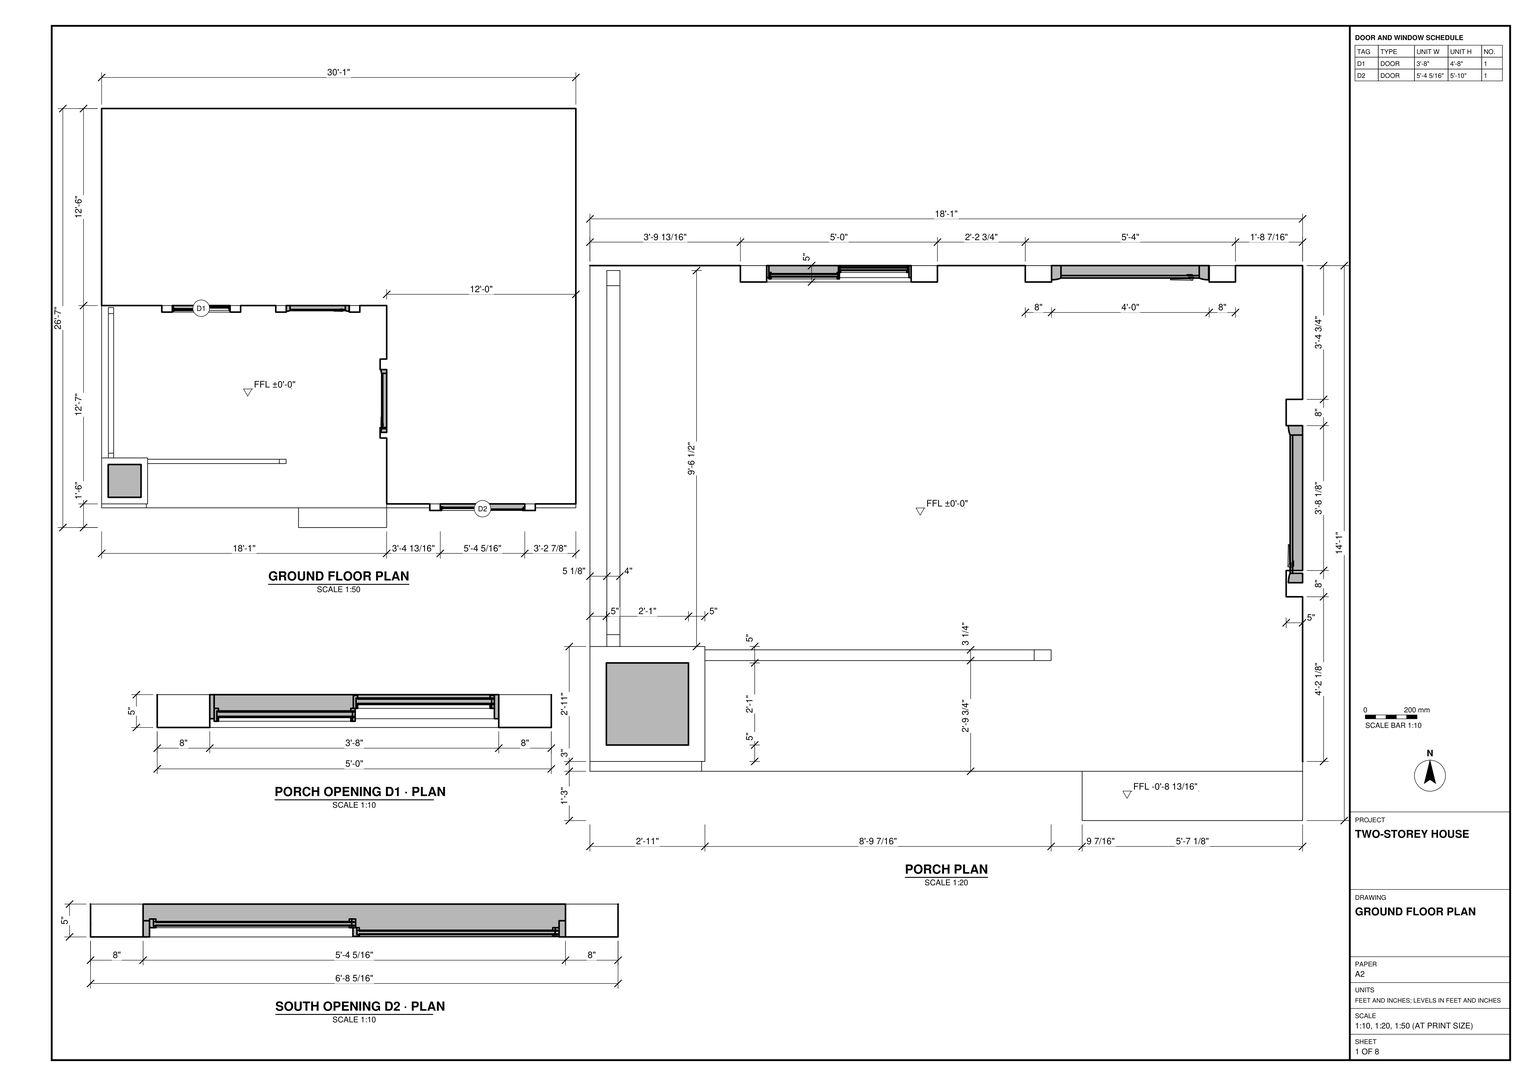
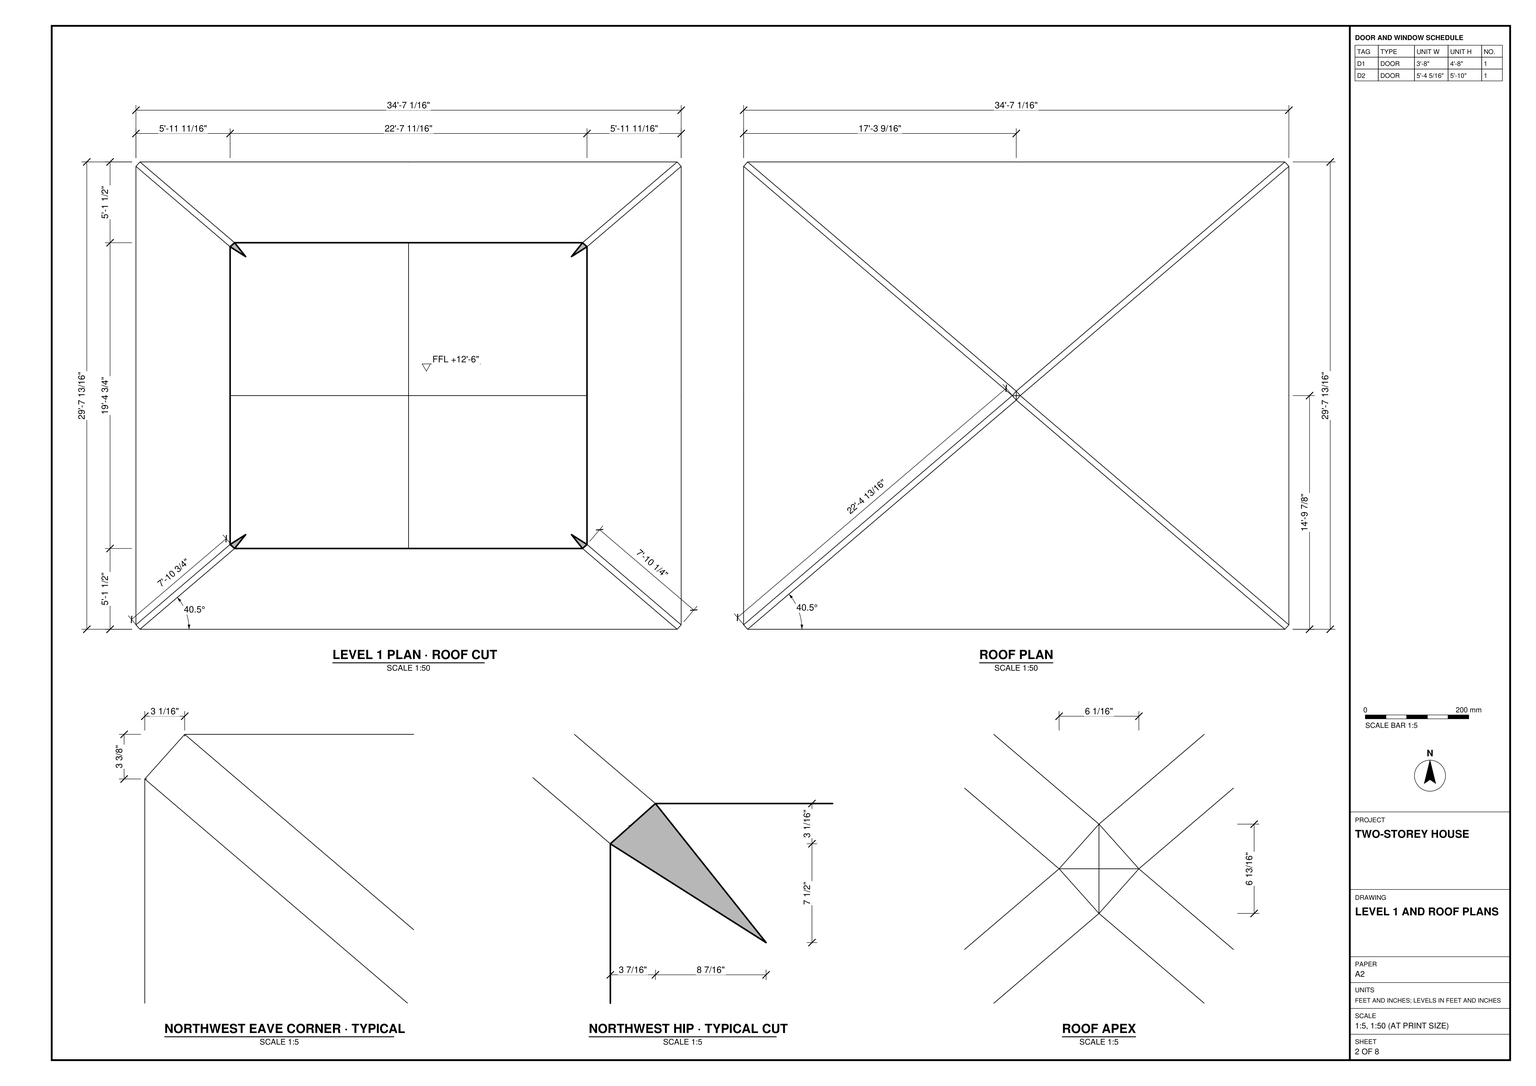
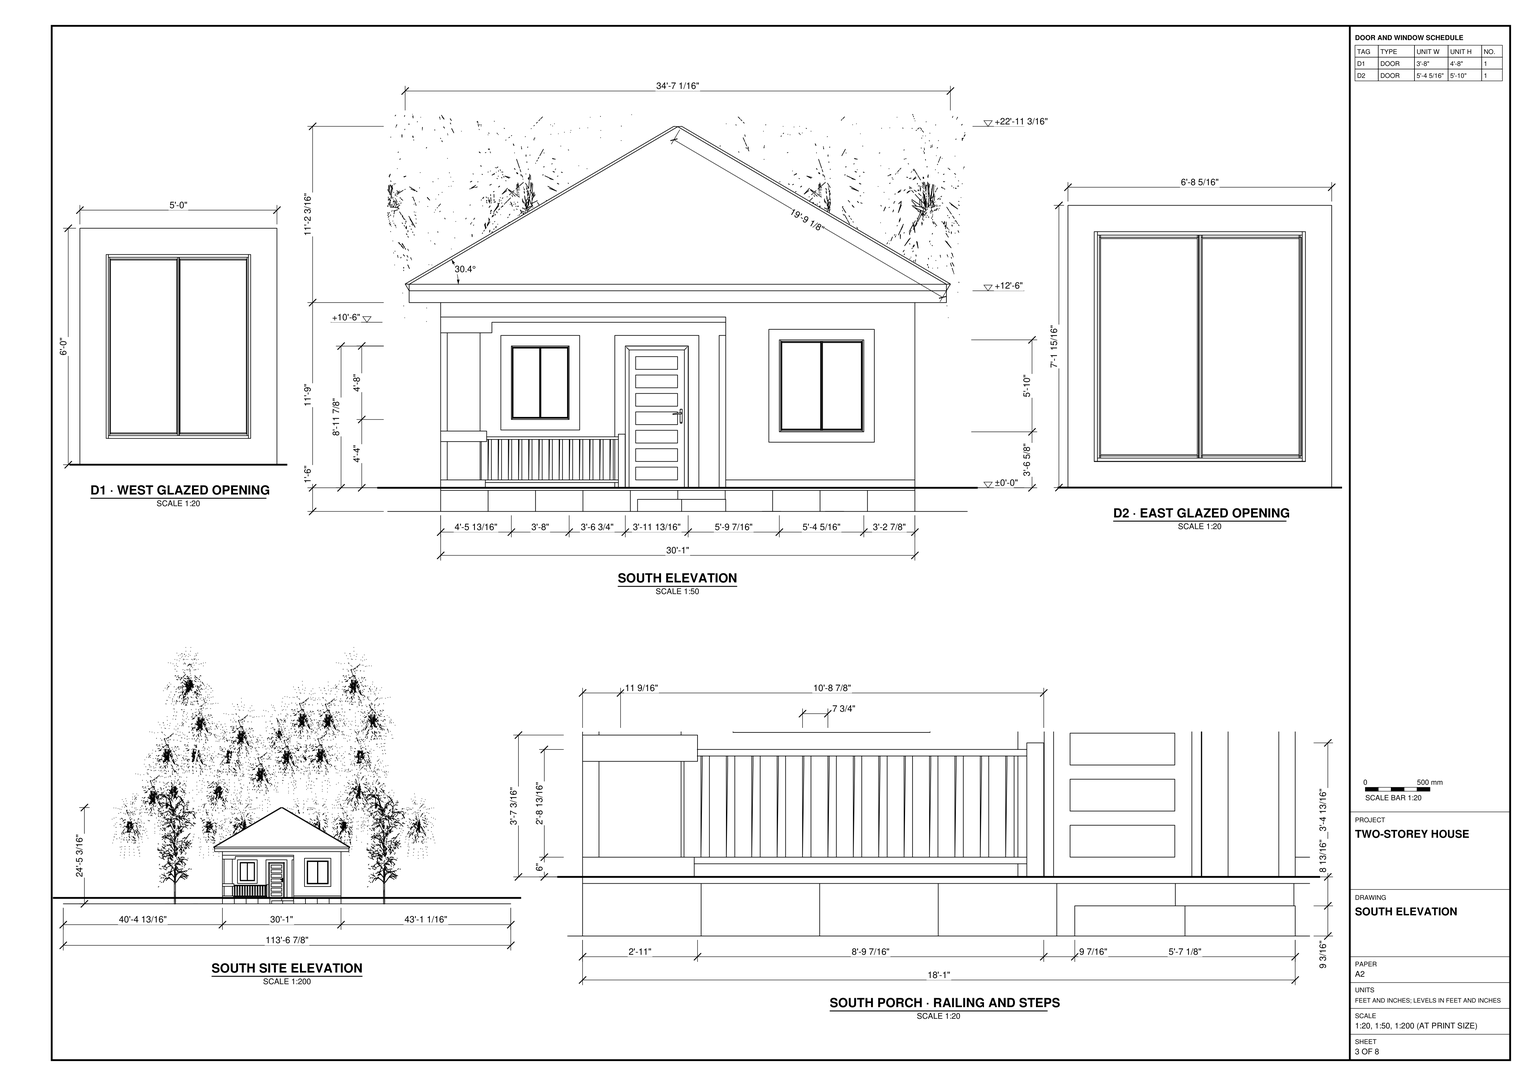
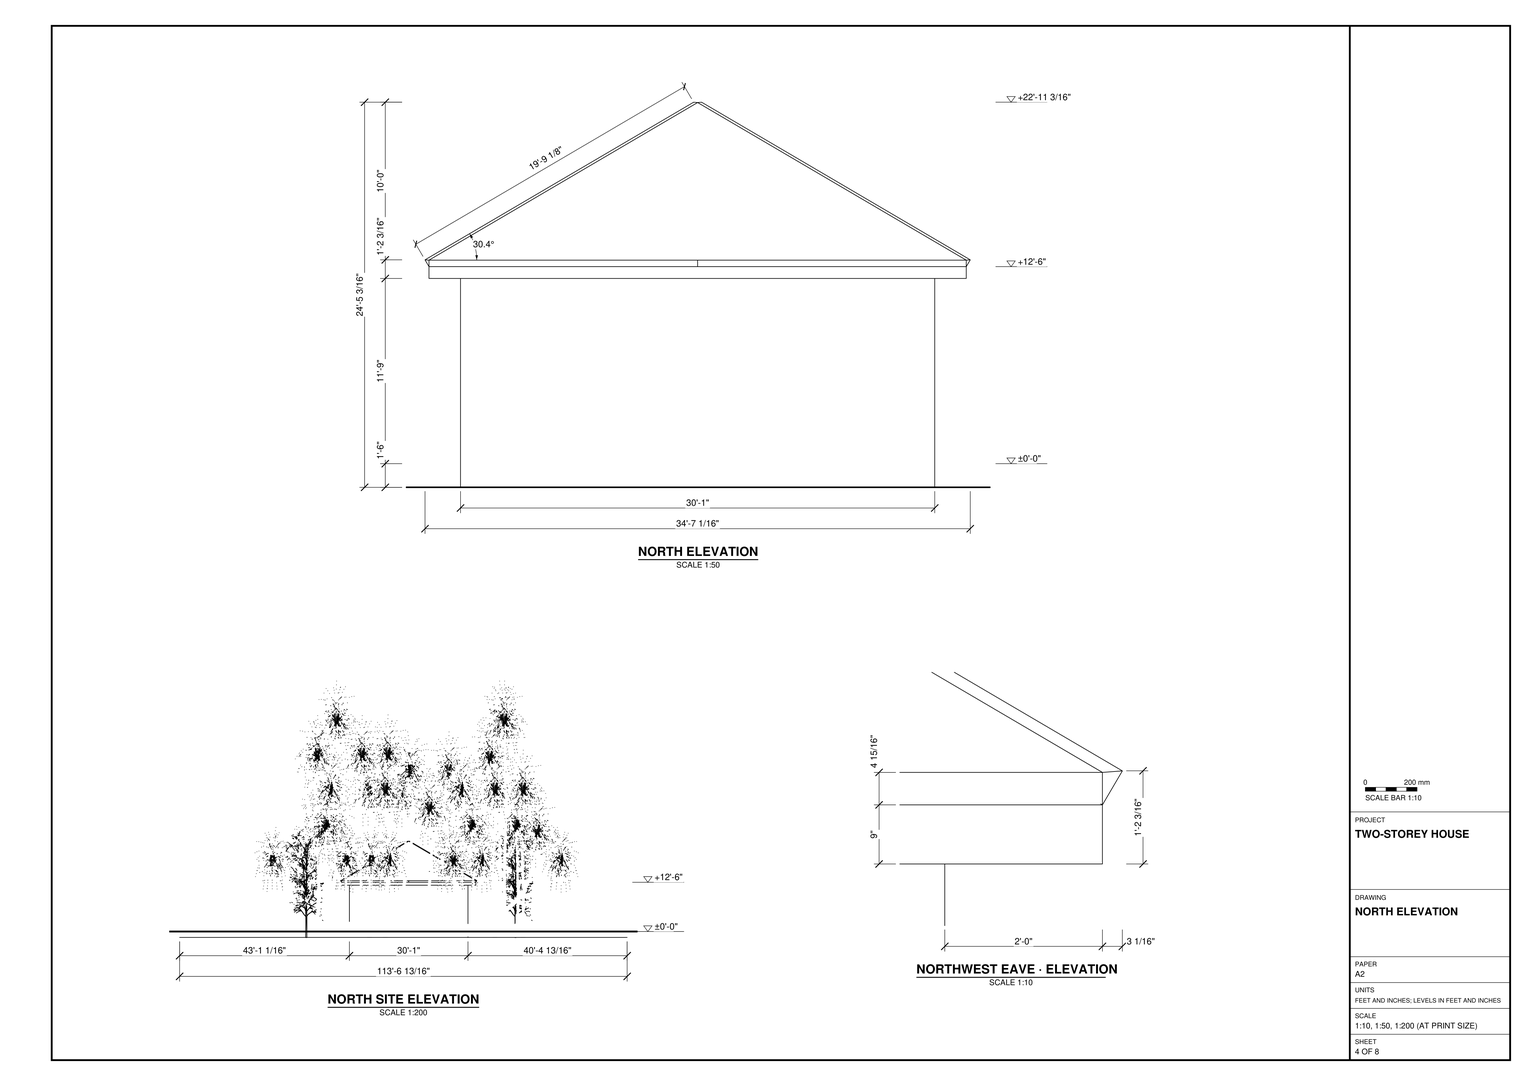
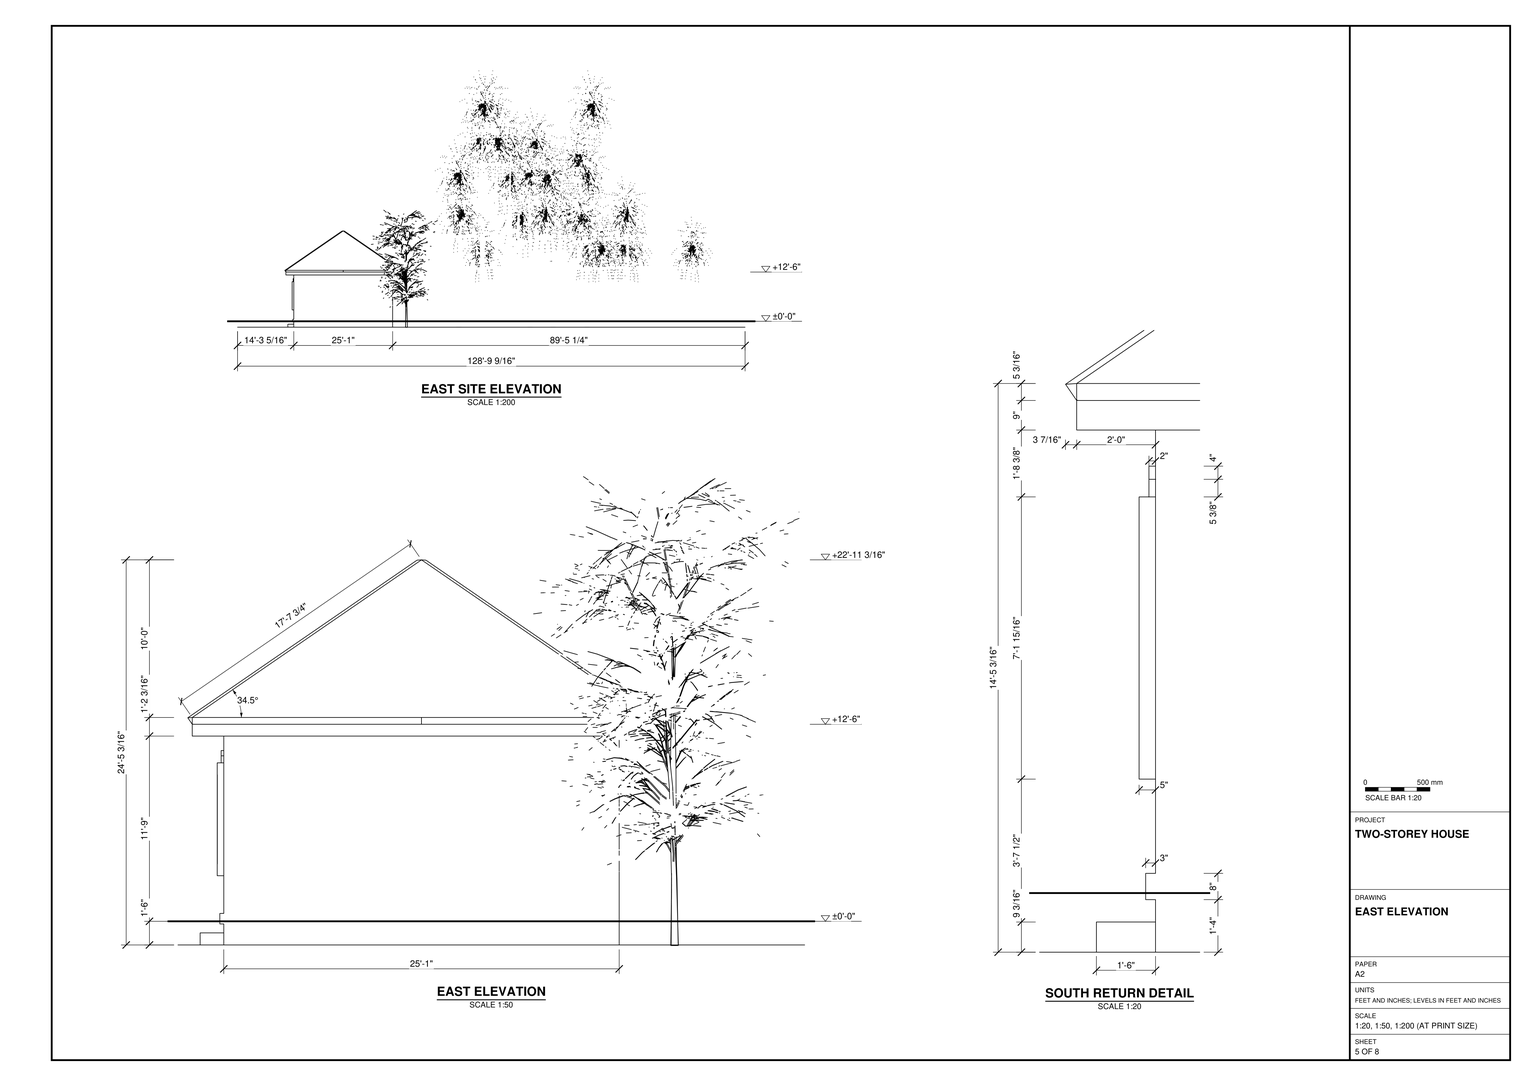
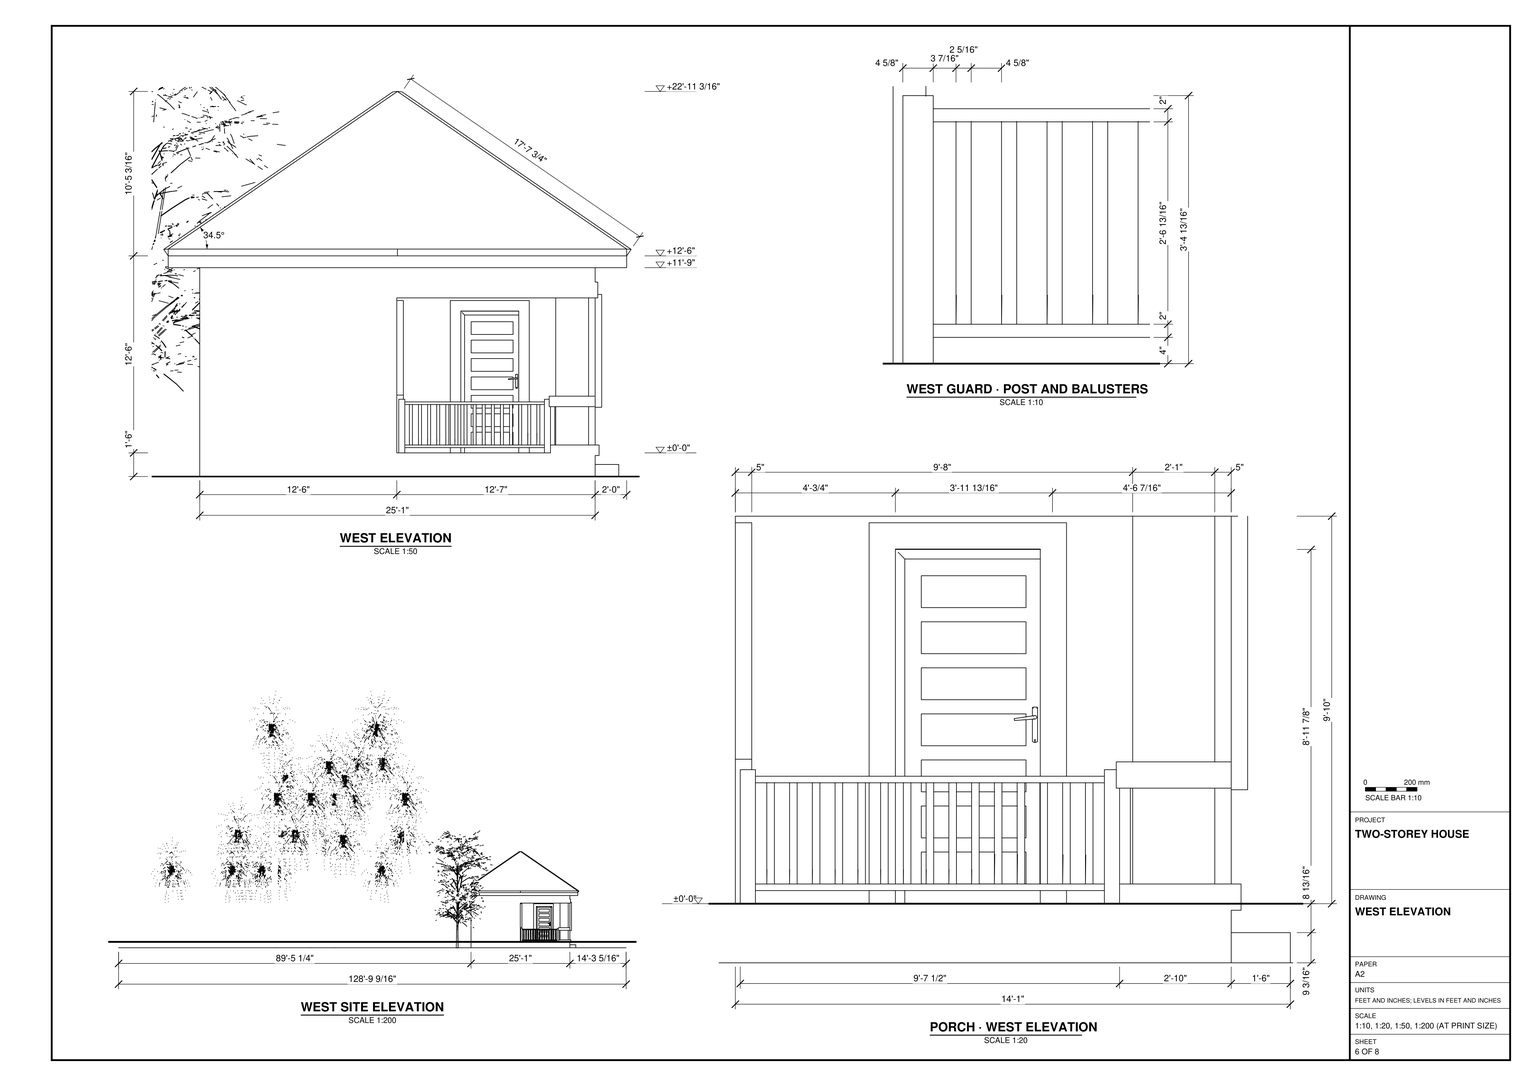
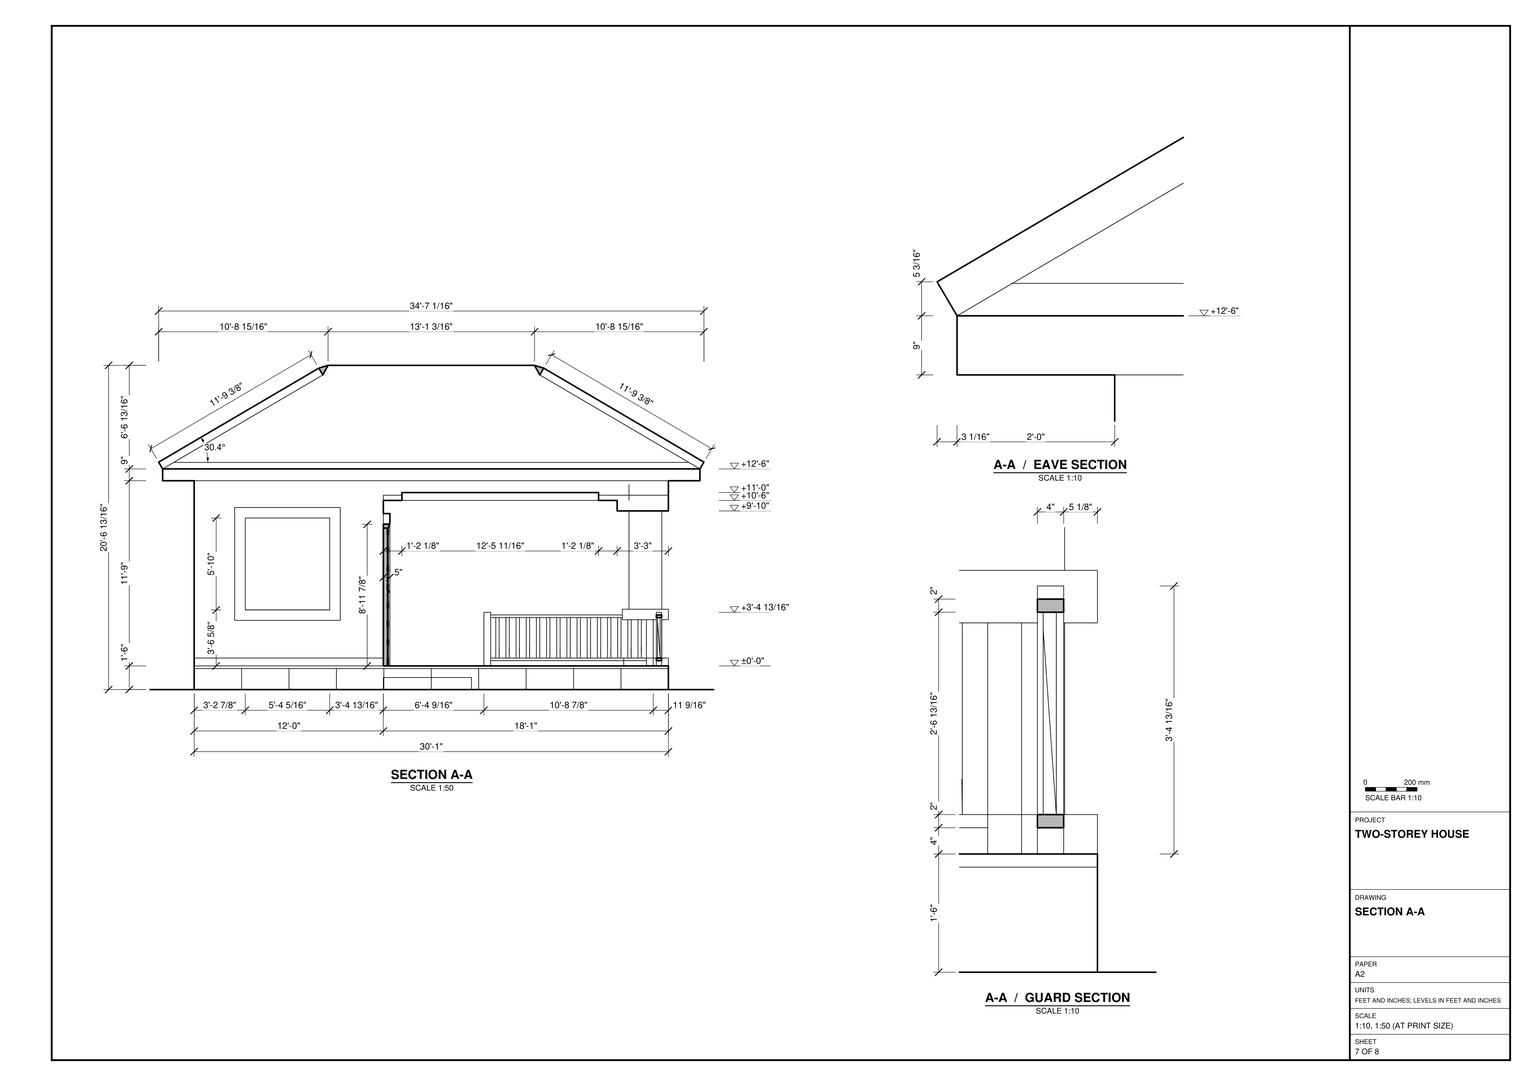
Build the house and its setting in SketchUp from task_files/diagram_01.pdf. Work in feet and inches. The complete model, including the site and planting, measures 113'-6 7/8" along X, 128'-9 9/16" along Y and 65'-6 1/2" along Z. Set the ground floor at ±0'-0" and the upper level at +12'-6".

Use the 30'-1" south frontage to lay out the house on its raised base. Follow the wall thicknesses and opening positions in plan. Recess the porch on the west part of the frontage, leaving the east part enclosed. Model the porch slab, entry steps, square corner support and railing, leaving a clear approach from the steps to the panelled entrance door. Fit the framed, two-panel glazed units into the walls, with the smaller unit at the back of the porch and the larger unit in the projecting south wall.

Use the upper-level roof cut and the roof plan to form four sloping faces that meet at a central apex. Carry the eaves beyond the walls and model the fascia shown in elevation. Include the trees around the house as shown in the site view. Planting, decor and loose items may be represented by any suitable library components.

Keep shell elements such as walls, slabs and roof, and each furniture or joinery piece shown, in separate groups or components. Use components for repeated parts. Save one SketchUp model as output_files/two_storey_house_with_a_recessed_porch_and_hipped_roof.skp.

# SketchUp Ruby script. Lengths in inches.
U = 1.inch
M = Sketchup.active_model
def pt(a) = Geom::Point3d.new(a.map { |v| v * U })
def face(e, loops, mat)
  f = e.add_face(loops[0].map { |a| pt(a) })
  loops[1..].each { |l| e.add_face(l.map { |a| pt(a) }).erase! }
  f.material = f.back_material = mat if mat
  f
end
# faces: each face lists its corners as indices into pts; further lists are holes
def faces(e, pts, list, mat = nil) = list.each { |f| face(e, (f[0].is_a?(Array) ? f : [f]).map { |l| l.map { |i| pts[i] } }, mat) }
# xy, xz, yz: faces in a plane at the given z, y or x. An outline is a flat list of corners, or four numbers for a rectangle; further outlines are holes
def ring(l) = l.size == 4 ? [[l[0], l[1]], [l[2], l[1]], [l[2], l[3]], [l[0], l[3]]] : l.each_slice(2).to_a
def flat(e, list, mat, &to3) = list.each { |f| face(e, (f[0].is_a?(Array) ? f : [f]).map { |l| ring(l).map { |u, v| to3.(u, v) } }, mat) }
def xy(e, z, list, mat = nil) = flat(e, list, mat) { |x, y| [x, y, z] }
def xz(e, y, list, mat = nil) = flat(e, list, mat) { |x, z| [x, y, z] }
def yz(e, x, list, mat = nil) = flat(e, list, mat) { |y, z| [x, y, z] }
def lines(e, pts, list) = list.each { |a, b| e.add_line(pt(pts[a]), pt(pts[b])) }
# prism: a flat outline (further loops are holes) pulled along v
def prism(e, loops, v, mat = nil)
  f = face(e, loops, mat); d = Geom::Vector3d.new(v.map { |x| x * U })
  f.pushpull(f.normal.samedirection?(d) ? d.length : -d.length)
end
def box(e, o, s, mat = nil) = prism(e, [[o, [o[0] + s[0], o[1], o[2]], [o[0] + s[0], o[1] + s[1], o[2]], [o[0], o[1] + s[1], o[2]]]], [0, 0, s[2]], mat)
def at(x, y, z, deg = 0) = Geom::Transformation.translation(pt([x, y, z])) * Geom::Transformation.rotation(ORIGIN, Z_AXIS, deg.degrees)
def axes(o, x, y, z) = Geom::Transformation.new([*x, 0, *y, 0, *z, 0, *pt(o).to_a, 1])
def part(name) = M.definitions.add(name)
# library, detail: a bought-in or finely detailed component or shape, given as its bounding box
def library(name, o, s) = part(name).tap { |d| box(d.entities, o, s) }
def detail(e, o, s) = box(e.add_group.entities, o, s)
def put(e, d, t, mat = nil) = e.add_instance(d, t).tap { |i| i.material = mat if mat }
def group(e, t, mat = nil) = e.add_group.tap { |g| g.transformation = t; g.material = mat if mat }.entities
root = M.entities
M.materials.add("COCOLUMBER1").color = [119, 109, 95]
M.materials.add("Glass_Tinted_Gray").color = [0, 0, 0]
M.materials["Glass_Tinted_Gray"].alpha = 0.125
M.materials.add("Wood_Grain_Dark").color = [94, 66, 25]
M.materials.add("[0049_Beige]").color = [245, 245, 220]
M.materials.add("[0135_DarkGray]").color = [81, 81, 81]
M.materials.add("[Granite Dark Gray]").color = [69, 68, 68]
M.materials.add("[Granite Tile]").color = [155, 148, 143]
M.materials.add("[Grass Dark Green]").color = [106, 157, 55]
M.materials.add("[Grass Light Green]").color = [138, 158, 69]
M.materials.add("[Mirror 02]").color = [229, 229, 229]
M.materials.add("[Roofing Tile Spanish]").color = [138, 64, 36]
M.materials.add("[Stone_Flagstone_Ashlar]").color = [175, 116, 102]
M.materials.add("[Terrazzo Light Blue]").color = [196, 214, 227]
c1 = part("PENTEK_RP Fineline 50S_Sliding_DoorCase_E1")
box(c1.entities,[0,0,0],[1.51,3.66,99.27],"[0135_DarkGray]")
c2 = part("PENTEK_RP Fineline 50S_SlidingDooe_Case_E2")
box(c2.entities,[0,0,0],[96.25,3.66,1.51],"[0135_DarkGray]")
c3 = part("pentek_RP Fineline 50S_SlidingDoor_Case")
put(c3.entities,c1,at(97.76,0,0))
put(c3.entities,c2,at(1.51,0,0))
put(c3.entities,c1,at(0,0,0))
put(c3.entities,c2,at(1.51,0,97.76))
c4 = part("PENTEK_RP Fineline 50S_SlidingDoor_GlazingBead_2")
box(c4.entities,[0,0,0],[0.56,0.59,94.39],"[0135_DarkGray]")
c5 = part("PENTEK_RP Fineline 50S_SlidingDoor_Glass")
box(c5.entities,[0,0,0],[46.58,0.16,94.39],"Glass_Tinted_Gray")
c6 = part("PENTEK_RP Fineline 50S_SlidingDoor_GlazingBead")
box(c6.entities,[0,0,0],[45.47,0.59,0.56],"[0135_DarkGray]")
c7 = part("PENTEK_RP Fineline 50S_SlidingDoor_Leaf_E1")
xy(c7.entities,0,[[0,0,0.93,1.97],[0.93,1.57,1.49,1.97]],"[0135_DarkGray]")
xy(c7.entities,96.25,[[0,0,0.93,0,0.93,1.57,1.49,1.57,1.49,1.97,0,1.97]],"[0135_DarkGray]")
xz(c7.entities,0,[[0,0,0.93,96.25]],"[0135_DarkGray]")
xz(c7.entities,1.57,[[0.93,0,1.49,95.32],[0.93,95.32,1.49,96.25]],"[0135_DarkGray]")
xz(c7.entities,1.97,[[0,0,1.49,96.25]],"[0135_DarkGray]")
yz(c7.entities,0,[[0,0,1.97,96.25]],"[0135_DarkGray]")
yz(c7.entities,0.93,[[0,0,1.57,0.93],[0,0.93,1.57,95.32],[0,95.32,1.57,96.25]],"[0135_DarkGray]")
yz(c7.entities,1.49,[[1.57,0,1.97,95.32],[1.57,95.32,1.97,96.25]],"[0135_DarkGray]")
c8 = part("PENTEK_RP Fineline 50S_SlidingDoor_Leaf_E2")
xy(c8.entities,0,[[0,0,0,1.57,0.56,1.57,0.56,1.97,46.02,1.97,46.02,1.57,46.58,1.57,46.58,0]],"[0135_DarkGray]")
xy(c8.entities,0.93,[[0,0,46.58,1.57]],"[0135_DarkGray]")
xy(c8.entities,1.49,[[0.56,1.57,46.02,1.97]],"[0135_DarkGray]")
xz(c8.entities,0,[[0,0,46.58,0.93]],"[0135_DarkGray]")
xz(c8.entities,1.57,[[0,0,0.56,0.93],[46.02,0,46.58,0.93],[0.56,0.93,46.02,1.49]],"[0135_DarkGray]")
xz(c8.entities,1.97,[[0.56,0,46.02,1.49]],"[0135_DarkGray]")
yz(c8.entities,0,[[0,0,1.57,0.93]],"[0135_DarkGray]")
yz(c8.entities,0.56,[[1.57,0,1.97,0.93],[1.57,0.93,1.97,1.49]],"[0135_DarkGray]")
yz(c8.entities,46.02,[[1.57,0,1.97,0.93],[1.57,0.93,1.97,1.49]],"[0135_DarkGray]")
yz(c8.entities,46.58,[[0,0,1.57,0.93]],"[0135_DarkGray]")
c9 = part("PENTEK_RP Fineline S_SlidingDoor_Leaf1")
put(c9.entities,c4,at(0.93,0,0.93))
put(c9.entities,c4,at(46.96,0,0.93))
put(c9.entities,c5,at(1.49,1.42,0.93))
put(c9.entities,c6,at(1.49,0,0.93))
put(c9.entities,c5,at(1.49,0.59,0.93),"[Terrazzo Light Blue]")
put(c9.entities,c7,at(0,0,0))
put(c9.entities,c7,axes([48.44,0,0],[-1,0,0],[0,1,0],[0,0,1]))
put(c9.entities,c8,axes([0.93,0,96.25],[1,0,0],[0,1,0],[0,0,-1]))
put(c9.entities,c8,at(0.93,0,0))
put(c9.entities,c6,at(1.49,0,94.77))
c10 = part("PENTEK_RP Fineline 50S_SlidingDoor_Leaf2")
put(c10.entities,c5,at(1.49,1.42,0.93))
put(c10.entities,c6,at(1.49,0,94.77))
put(c10.entities,c4,at(46.96,0,0.93))
put(c10.entities,c5,at(1.49,0.59,0.93),"[Mirror 02]")
put(c10.entities,c4,at(0.93,0,0.93))
put(c10.entities,c7,at(0,0,0))
put(c10.entities,c7,axes([48.44,0,0],[-1,0,0],[0,1,0],[0,0,1]))
put(c10.entities,c6,at(1.49,0,0.93))
put(c10.entities,c8,axes([0.93,0,96.25],[1,0,0],[0,1,0],[0,0,-1]))
put(c10.entities,c8,at(0.93,0,0))
c11 = part("PENTEK - Slimmest Steel Sliding Door / Window\#1")
put(c11.entities,c3,at(0,-1.88,-0.09))
put(c11.entities,c9,at(1.51,-2.27,1.42))
put(c11.entities,c10,at(49.32,-0.3,1.42))
c12 = library("Untitled (4)",[17.32,30.71,0],[35.44,8.12,78.74])
c13 = part("railing post")
xy(c13.entities,0,[[0,0,2,2]],"Wood_Grain_Dark")
xy(c13.entities,31,[[0,0,2,0,2,2,0.3125,2]],"Wood_Grain_Dark")
xz(c13.entities,0,[[0,0,2,31]],"Wood_Grain_Dark")
xz(c13.entities,2,[[0,0,0.3125,28.1875,0.3125,31,2,31,2,0]],"Wood_Grain_Dark")
yz(c13.entities,2,[[0,0,2,31]],"Wood_Grain_Dark")
p = [[0.3125,2,28.1875],[0,2,0],[0,0,0],[0,0,31],[0.3125,2,31]]
faces(c13.entities,p,[[0,1,2],[0,2,3,4]],"Wood_Grain_Dark")
c14 = part("cgb5189+Railing+sketch+up")
put(c14.entities,c13,at(60.61,35.39,6))
put(c14.entities,c13,at(66.61,35.39,6))
put(c14.entities,c13,at(72.61,35.39,6))
put(c14.entities,c13,at(78.61,35.39,6))
put(c14.entities,c13,at(84.61,35.39,6))
put(c14.entities,c13,at(90.61,35.39,6))
put(c14.entities,c13,at(96.61,35.39,6))
put(c14.entities,c13,at(102.61,35.39,6))
put(c14.entities,c13,at(54.61,35.39,6))
put(c14.entities,c13,at(48.61,35.39,6))
put(c14.entities,c13,at(42.61,35.39,6))
put(c14.entities,c13,at(36.61,35.39,6))
put(c14.entities,c13,at(30.61,35.39,6))
put(c14.entities,c13,at(24.61,35.39,6))
put(c14.entities,c13,at(18.61,35.39,6))
g1 = group(c14.entities,at(11.61,34.27,0))
box(g1,[0,0,0],[4,4,40.8125],"Wood_Grain_Dark")
g2 = group(c14.entities,at(15.61,34.27,4))
box(g2,[0,0,0],[92,4,2],"Wood_Grain_Dark")
g3 = group(c14.entities,at(15.61,34.27,36.8125))
xy(g3,0,[[0,0,92,4]],"Wood_Grain_Dark")
xy(g3,2,[[0,0,92,4]],"Wood_Grain_Dark")
xz(g3,0,[[0,0,92,2]],"Wood_Grain_Dark")
xz(g3,4,[[0,0,92,2]],"Wood_Grain_Dark")
yz(g3,0,[[0,0,4,2]])
yz(g3,92,[[0,0,4,2]])
g4 = group(c14.entities,at(107.61,34.27,0))
box(g4,[0,0,0],[4,4,40.8125],"Wood_Grain_Dark")
c15 = library("Palm frond",[-21.27,-0.38,-4.44],[74.64,151.68,26.05])
c16 = part("Palm frond cluster")
put(c16.entities,c15,axes([98.98,59.12,-6.6],[-0.57786,0.81614,0],[-0.81614,-0.57786,0],[0,0,1.8876]))
put(c16.entities,c15,axes([105.83,88.13,9.87],[-0.67944,-0.73373,0],[0.7249,-0.67126,-0.15471],[0.21427,-0.19842,1.86487]))
put(c16.entities,c15,axes([73.46,76.73,-6.83],[1,0,0],[0,0.99443,-0.10543],[0,0.19901,1.87708]))
c17 = part("Palm tree")
put(c17.entities,c15,axes([108.09,116.23,112.23],[0.60444,0.79634,0.02211],[-0.38669,0.31755,-0.86581],[-0.57427,0.42444,0.41215]))
put(c17.entities,c15,axes([136.99,132.05,110.62],[-0.9152,-0.38852,0.10706],[0.08408,-0.44389,-0.89213],[0.32496,-0.66577,0.36188]))
put(c17.entities,c15,axes([122.18,113.8,111.54],[0.08804,0.99481,0.05098],[-0.50379,0.08862,-0.85927],[-0.70852,0.0412,0.41966]))
put(c17.entities,c15,axes([127.99,125.91,114.12],[-0.30715,0.21543,0.04369],[-0.00716,-0.23041,1.0858],[0.26841,0.36655,0.07955]))
put(c17.entities,c15,axes([103.59,126.54,118.32],[0.96893,0.24682,0.01605],[-0.22321,0.84461,0.48663],[0.20112,-0.89679,1.64874]))
put(c17.entities,c15,axes([132.625,118.58,110.86],[-0.79198,0.60227,0.10017],[-0.36651,-0.33776,-0.86694],[-0.4026,-0.59638,0.40255]))
put(c17.entities,c15,axes([132.69,143.375,115.86],[-0.48474,-0.87071,0.083],[0.68927,-0.43869,-0.5766],[1.01639,-0.4196,1.53425]))
put(c17.entities,c16,axes([128.89,9.89,132.21],[0.59014,0.791,-0.16144],[-0.79634,0.60321,0.04452],[0.1326,0.10229,0.98588]))
put(c17.entities,c15,axes([110.58,141.22,117.1],[0.63855,-0.76931,0.0202],[0.63758,0.51415,-0.57371],[0.8135,0.71582,1.54559]))
put(c17.entities,c15,axes([124.78,146.64,115.88],[-0.11221,-0.99112,0.07129],[0.92652,-0.13028,-0.35296],[0.67787,0.04993,1.76097]))
put(c17.entities,c15,axes([122.51,149.42,117.04],[0.39103,-0.91975,0.03404],[0.19966,0.04866,-0.97866],[0.74078,0.32113,0.1671]))
put(c17.entities,c15,axes([109.625,140.35,117.99],[0.86054,-0.50891,0.02211],[0.4462,0.77402,0.44921],[-0.46382,-0.71105,1.68592]))
put(c17.entities,c15,axes([116.71,128.1875,118.1],[0.61604,-0.07661,0.00027],[0.03235,0.25679,-0.96593],[0.09819,0.79033,0.2134]),"COCOLUMBER1")
put(c17.entities,c15,axes([106.79,121.78,118.63],[0.90526,0.41496,-0.09122],[-0.38356,0.70587,-0.59551],[-0.34491,1.08363,1.50659]))
put(c17.entities,c15,axes([127.38,115.49,111.15],[-0.41996,0.90406,0.07938],[-0.48716,-0.15078,-0.8602],[-0.63133,-0.32974,0.41534]))
put(c17.entities,c15,axes([126.87,112.82,117.51],[-0.39428,0.9188,-0.01857],[-0.74747,-0.33238,-0.57517],[-1.00919,-0.40185,1.54373]))
put(c17.entities,c15,axes([136.51,114.68,116.54],[-0.8132,0.57038,0.11567],[-0.44883,-0.74115,0.49924],[0.69933,0.66833,1.62089]))
put(c17.entities,c15,axes([139.34,132.85,114.96],[-0.95658,-0.27018,0.10937],[0.1925,-0.86734,-0.45898],[0.41314,-0.78901,1.66428]))
put(c17.entities,c15,axes([114.58,111.42,117.76],[0.273,0.96044,0.05495],[-0.82871,0.20578,0.52048],[0.92224,-0.35418,1.60843]))
put(c17.entities,c16,axes([34.06,50.17,99.19],[1,0,0],[0,0.96593,0.25882],[0,-0.25882,0.96593]))
put(c17.entities,c15,axes([129.57,143.93,113.7],[-0.59821,-0.79634,0.08934],[0.41703,-0.40458,-0.81388],[0.56418,-0.37071,0.47337]))
put(c17.entities,c15,axes([130.72,144.4375,116.95],[-0.38164,-0.91976,0.09155],[0.8496,-0.31006,0.42666],[-0.68716,0.45418,1.6984]))
put(c17.entities,c15,axes([131.04,111.78,119.35],[-0.80044,0.5994,0.00413],[-0.42618,-0.56425,-0.7071],[-0.79563,-1.07169,1.33472]))
put(c17.entities,c15,axes([110.2,144.05,126.35],[0.60643,-0.7943,0.03632],[0.64903,0.52087,0.55448],[-0.86705,-0.59022,1.56936]))
put(c17.entities,c15,axes([142.64,131.42,116.29],[-0.95847,-0.25692,0.12379],[0.28487,-0.84195,0.45823],[-0.02548,0.8956,1.66141]))
put(c17.entities,c15,axes([119.45,118.27,117.33],[0.21648,0.59293,0.03228],[-0.46829,0.12335,0.87492],[0.90601,-0.35995,0.53567]))
put(c17.entities,c15,axes([117.27,113.7,118.04],[0.23506,0.97049,-0.05375],[-0.80388,0.16302,-0.57201],[-1.03133,0.33537,1.54496]))
put(c17.entities,c15,axes([111.15,130.86,117.79],[0.59448,-0.21434,0.01115],[0.17045,0.51639,0.83922],[-0.32671,-0.8747,0.60458]))
put(c17.entities,c15,axes([131.22,120.64,116.67],[-0.51397,0.3605,0.07311],[-0.2051,-0.46687,0.86021],[0.60585,0.75173,0.55245]))
put(c17.entities,c15,axes([124.93,138.67,117.02],[-0.21153,-0.59293,0.0562],[0.56288,-0.12335,0.81728],[-0.84066,0.35995,0.63331]))
put(c17.entities,c15,axes([125.97,109.88,116.19],[-0.24621,0.96375,0.10281],[-0.94431,-0.21463,-0.24942],[-0.41209,-0.29916,1.81761]))
put(c17.entities,c15,axes([112.49,114.18,118.67],[0.68775,0.72163,-0.07906],[-0.67912,0.60109,-0.4213],[-0.48416,0.64828,1.70539]))
c18 = part("Group\#111")
put(c18.entities,c17,axes([-0.04,31.24,176.27],[0.54092,-0.14494,0],[0.14494,0.54092,0],[0,0,0.56]),"[Stone_Flagstone_Ashlar]")
g5 = group(c18.entities,at(43.85,611.85,9.84))
detail(g5,[29.01,-534.03,-9.84],[20.18,17.89,236.22])
c19 = library("Group\#103",[280.3,-607.43,-9.84],[21.76,21.76,393.7])
c20 = part("Group\#116")
put(c20.entities,c17,axes([14.65,13.97,332.76],[0.56,0,0],[0,0.56,0],[0,0,0.56]),"[Stone_Flagstone_Ashlar]")
put(c20.entities,c19,at(-205.96,691.71,9.84))
c21 = library("Group\#102",[336.49,-607.32,-9.84],[23.63,23.62,472.44])
c22 = part("Group\#117")
put(c22.entities,c17,axes([14.65,13.97,408.41],[0.56,0,0],[0,0.56,0],[0,0,0.56]),"[Stone_Flagstone_Ashlar]")
put(c22.entities,c21,axes([-199.25,630.26,9.84],[0.8099,0,0],[0,0.92,0],[0,0,1]))
c23 = part("Group\#13")
put(c23.entities,c17,axes([14.65,13.97,257.21],[0.56,0,0],[0,0.56,0],[0,0,0.56]),"[Stone_Flagstone_Ashlar]")
g6 = group(c23.entities,at(-87.26,634.75,9.84))
detail(g6,[163.83,-557.35,-9.84],[17.02,18.12,316.37])
c24 = library("Coconut",[0,0,0],[6,6,6])
c25 = part("Group\#106")
detail(c25.entities,[126.53,-566.4375,-31.76],[21.43,21.47,314.96])
c26 = part("Group\#109")
put(c26.entities,c17,axes([14.65,13.97,253.0625],[0.56,0,0],[0,0.56,0],[0,0,0.56]),"[Stone_Flagstone_Ashlar]")
put(c26.entities,c25,at(-54.86,642.08,31.76))
c27 = library("Group\#349",[-31.7,-22.28,0],[197.44,197.48,245.38])
c28 = library("Group\#217",[-86.05,-583.93,-9.84],[105.44,25.13,372.44])
c29 = part("Group\#229")
put(c29.entities,c17,axes([14.65,13.97,296.01],[0.56,0,0],[0,0.56,0],[0,0,0.56]),"[Stone_Flagstone_Ashlar]")
put(c29.entities,c28,axes([86.81,656.51,9.45],[1,0,0],[0,1,0],[0,0,0.96]))
c30 = library("Group\#220",[-509.61,-583,-9.84],[198.33,25,224.95])
c31 = part("Group\#226")
put(c31.entities,c17,axes([14.65,13.97,164.57],[0.56,0,0],[0,0.56,0],[0,0,0.56]),"[Stone_Flagstone_Ashlar]")
put(c31.entities,c30,at(588.97,655.37,9.84))
c32 = library("Group\#218",[-201.8,-584.81,-9.84],[84.72,26.88,386.61])
c33 = library("Group\#219",[-284.02,-582.12,-9.84],[34.81,21.51,275.59])
c34 = part("LANDSCAPING+Coconut+Trees")
xy(c34.entities,0,[[-341.57,-22.89,1280.875,1071.24]],"[Grass Light Green]")
put(c34.entities,c18,at(644.25,162.65,0.08,-90))
put(c34.entities,c20,at(534.68,153.22,0.24))
put(c34.entities,c22,at(627.57,68.88,0.24))
g7 = group(c34.entities,at(441.06,62.32,0.24))
put(g7,c17,axes([14.65,13.97,334.3],[0.56,0,0],[0,0.56,0],[0,0,0.56]),"[Stone_Flagstone_Ashlar]")
g8 = group(g7,at(-161.71,683.51,9.84))
detail(g8,[235.77,-605.36,-9.84],[21.85,21.73,393.32])
put(c34.entities,c23,at(507.45,-17.04,0.04))
g9 = group(c34.entities,at(384.92,163.75,0.52))
put(g9,c17,axes([14.65,13.97,253.0625],[0.56,0,0],[0,0.56,0],[0,0,0.56]),"[Stone_Flagstone_Ashlar]")
put(g9,c24,axes([78.15,82.49,296.44],[0.8993,1.53487,-0.03138],[-1.51998,0.89531,0.23158],[0.21557,-0.09025,1.76378]))
put(g9,c24,axes([79.68,82.54,287.24],[0.80142,1.36782,-0.02796],[-1.35455,0.79787,0.20637],[0.1921,-0.08042,1.57182]))
put(g9,c24,axes([77.51,71.8,291.02],[0.8993,1.53487,-0.03138],[-1.51998,0.89531,0.23158],[0.21557,-0.09025,1.76378]))
put(g9,c24,axes([86.52,87.55,293.71],[1.04679,1.7866,-0.03652],[-1.76927,1.04215,0.26956],[0.25092,-0.10505,2.05306]))
put(g9,c24,axes([92.01,70.93,291.34],[1.26662,2.16178,-0.04419],[-2.14081,1.261,0.32616],[0.30361,-0.12711,2.4842]))
put(g9,c25,at(-54.86,642.08,31.76))
put(c34.entities,c26,at(322.43,275.42,0.52,75))
put(c34.entities,c27,at(215.66,444.05,0))
put(c34.entities,c29,at(219.87,194.55,1.28))
put(c34.entities,c31,at(-99.86,200.06,0.67))
g10 = group(c34.entities,at(71.46,249.51,0.63))
put(g10,c17,axes([14.65,13.97,325.99],[0.56,0,0],[0,0.56,0],[0,0,0.56]),"[Stone_Flagstone_Ashlar]")
put(g10,c32,at(259.05,660.06,9.84))
g11 = group(c34.entities,at(290.4,300.18,0.67))
put(g11,c17,axes([14.65,13.97,214.81],[0.56,0,0],[0,0.56,0],[0,0,0.56]),"[Stone_Flagstone_Ashlar]")
put(g11,c33,at(354.13,659.23,9.84))
put(c34.entities,c27,at(768.63,688.84,0,159))
put(c34.entities,c27,at(573.53,797.54,0,75))
put(c34.entities,c22,at(18.43,450.01,0.24))
put(c34.entities,c20,at(864.55,292.18,0.24,180))
put(c34.entities,c18,at(695.7,287.05,0.08))
put(c34.entities,c18,at(135.65,408.5625,0.08))
put(c34.entities,c31,at(771.29,622.71,0.67,-134.5))
put(c34.entities,c18,at(664.4,571.51,0.08))
put(c34.entities,c29,at(563.8125,499.28,1.28,140.1))
put(c34.entities,c23,at(450.29,232.17,0.04))
put(c34.entities,c23,at(-49.04,312.68,0.04))
put(c34.entities,c23,at(52.82,431.375,0.04))
put(c34.entities,c27,at(259.5,238.44,0,-105))
put(c34.entities,c27,at(533.19,658.43,0,-105))
put(c34.entities,c18,at(-26.35,370.51,0.08))
put(c34.entities,c27,at(-48.71,797.54,0,75))
put(c34.entities,c27,at(238.42,585.39,0,75))
put(c34.entities,c27,at(891.93,658.43,0,-105))
put(c34.entities,c22,at(220.5,234.49,0.24,165))
put(c34.entities,c26,at(795.86,275.42,0.52,75))
c35 = library("GoldenBamboo",[-21.19,-21.7,-0.46],[44.22,41.02,72.81])
xy(root,0,[[634.67,153.3125,701.8,171.3125],[484.8,171.3125,845.8,472.3125]])
xy(root,0,[[[613.89,0,613.89,132.875,440.09,132.875,440.09,597.94,860.62,597.94,860.62,132.875,713.38,132.875,713.38,0],[634.67,153.3125,701.8,153.3125,701.8,171.3125,845.8,171.3125,845.8,472.3125,484.8,472.3125,484.8,171.3125,634.67,171.3125]]],"[Granite Tile]")
xy(root,0,[[0,0,0,593.64,341.57,593.64,341.57,597.94,440.09,597.94,440.09,132.875,613.89,132.875,613.89,0],[713.38,0,713.38,132.875,860.62,132.875,860.62,597.94,924.05,597.94,924.05,593.64,1362.85,593.64,1362.85,0]],"[Grass Dark Green]")
xy(root,9.1875,[[634.67,153.3125,701.8,171.3125]],"[Granite Dark Gray]")
xy(root,16,[[484.8,168.3125,518.8,171.3125],[518.8,168.3125,701.8,171.3125],[701.8,168.3125,845.8,171.3125]],"[0049_Beige]")
xy(root,18,[[617.36,317.3125,625.36,322.3125],[673.36,317.3125,681.36,322.3125]])
xy(root,18,[[518.8,168.3125,701.8,168.3125,701.8,221.46,696.8,221.46,696.8,229.46,701.8,229.46,701.8,273.57,696.8,273.57,696.8,281.57,701.8,281.57,701.8,322.3125,681.36,322.3125,681.36,317.3125,673.36,317.3125,673.36,322.3125,625.36,322.3125,625.36,317.3125,617.36,317.3125,617.36,322.3125,484.8,322.3125,484.8,205.3125,518.8,205.3125]],"[Granite Dark Gray]")
xy(root,24,[[[484.8,168.3125,518.8,205.3125],[489.8,176.3125,514.8,201.3125]],[701.8,168.3125,845.8,171.3125]],"[0049_Beige]")
xy(root,52.7,[[734.61,166.3125,814.92,171.3125]])
xy(root,53.1875,[[489.8,176.3125,514.8,201.3125]])
xy(root,53.1875,[[484.8,171.3125,519.8,176.3125],[484.8,176.3125,489.8,206.3125],[514.8,176.3125,519.8,206.3125],[489.8,201.3125,514.8,206.3125]],"[0049_Beige]")
xy(root,60.7,[[742.61,166.3125,806.92,171.3125]],"[0049_Beige]")
xy(root,61.1875,[[489.8,176.3125,514.8,201.3125]])
xy(root,61.1875,[[[484.8,171.3125,519.8,206.3125],[489.8,176.3125,514.8,201.3125]]],"[0049_Beige]")
xy(root,62,[[530.61,317.3125,590.61,322.3125]])
xy(root,70,[[538.61,317.3125,582.61,322.3125]],"[0049_Beige]")
xy(root,126,[[538.61,317.3125,582.61,322.3125]])
xy(root,126,[[696.8,229.46,701.8,273.57],[625.36,317.3125,673.36,322.3125]],"[0049_Beige]")
xy(root,130.64,[[742.61,166.3125,806.92,171.3125]])
xy(root,134,[[696.8,221.46,701.8,281.57],[530.61,317.3125,590.61,322.3125],[617.36,317.3125,681.36,322.3125]],"[0049_Beige]")
xy(root,136,[[489.8,176.3125,514.8,201.3125]])
xy(root,136,[[[484.8,169.3125,523.8,322.3125],[489.8,176.3125,514.8,201.3125]]],"[0049_Beige]")
xy(root,138.64,[[734.61,166.3125,814.92,171.3125]],"[0049_Beige]")
xy(root,144,[[[523.8,169.3125,701.8,322.3125],[537.95,183.46,687.65,308.17]]],"[0049_Beige]")
xy(root,148,[[484.8,169.3125,514.8,171.3125],[514.8,169.3125,701.8,171.3125]])
xy(root,150,[[537.95,183.46,687.65,308.17]],"[0049_Beige]")
xy(root,159,[[460.8,147.3125,869.8,171.3125],[460.8,171.3125,484.8,496.3125],[845.8,171.3125,869.8,496.3125],[484.8,472.3125,845.8,496.3125]],"[0049_Beige]")
xy(root,168,[[460.8,147.3125,665.3,321.8125],[665.3,147.3125,869.8,321.8125],[460.8,321.8125,665.3,496.3125],[665.3,321.8125,869.8,496.3125]])
xz(root,147.3125,[[460.8,159,869.8,168]],"[0049_Beige]")
xz(root,153.3125,[[634.67,0,668.24,9.1875],[668.24,0,701.8,9.1875]],"[Granite Dark Gray]")
xz(root,166.3125,[[[734.61,52.7,814.92,138.64],[742.61,60.7,806.92,130.64]]],"[0049_Beige]")
xz(root,168.3125,[[701.8,18,845.8,24]],"[0049_Beige]")
xz(root,168.3125,[[484.8,16,845.8,16,845.8,18,518.8,18,518.8,24,484.8,24]],"[Granite Dark Gray]")
xz(root,169.3125,[[484.8,136,523.8,136,523.8,144,701.8,144,701.8,148,484.8,148]],"[0049_Beige]")
xz(root,171.3125,[[634.67,0,665.3,9.1875],[665.3,0,701.4,9.1875],[701.4,0,701.8,9.1875],[742.61,60.7,806.92,130.64]])
xz(root,171.3125,[[[701.8,24,845.8,24,845.8,159,484.8,159,484.8,148,701.8,148],[734.61,52.7,814.92,138.64]],[484.8,53.1875,519.8,61.1875]],"[0049_Beige]")
xz(root,171.3125,[[484.8,0,520.9,16],[520.9,0,557,16],[557,0,593.1,16],[593.1,0,629.2,16],[629.2,0,634.67,0,634.67,9.1875,665.3,9.1875,665.3,16,629.2,16],
  [701.8,0,737.5,0,737.5,16,701.4,16,701.4,9.1875,701.8,9.1875],[737.5,0,773.6,16],[773.6,0,809.7,16],[809.7,0,845.8,16],[665.3,9.1875,701.4,16]],"[Granite Dark Gray]")
xz(root,176.3125,[[489.8,24,514.8,53.1875],[489.8,61.1875,514.8,136]],"[0049_Beige]")
xz(root,183.46,[[537.95,144,687.65,150]],"[0049_Beige]")
xz(root,201.3125,[[489.8,24,514.8,53.1875],[489.8,61.1875,514.8,136]],"[0049_Beige]")
xz(root,205.3125,[[484.8,18,518.8,24]],"[0049_Beige]")
xz(root,206.3125,[[484.8,53.1875,519.8,61.1875]],"[0049_Beige]")
xz(root,221.46,[[696.8,18,701.8,134]],"[0049_Beige]")
xz(root,229.46,[[696.8,18,701.8,126]],"[0049_Beige]")
xz(root,273.57,[[696.8,18,701.8,126]],"[0049_Beige]")
xz(root,281.57,[[696.8,18,701.8,134]],"[0049_Beige]")
xz(root,308.17,[[537.95,144,687.65,150]],"[0049_Beige]")
xz(root,317.3125,[[617.36,18,625.36,18,625.36,126,673.36,126,673.36,18,681.36,18,681.36,134,617.36,134],[[530.61,62,590.61,134],[538.61,70,582.61,126]]],"[0049_Beige]")
xz(root,322.3125,[[617.36,10,681.36,18],[625.36,18,673.36,126],[538.61,70,582.61,126]])
xz(root,322.3125,[[[484.8,18,617.36,18,617.36,134,681.36,134,681.36,18,701.8,18,701.8,144,523.8,144,523.8,136,484.8,136],[530.61,62,590.61,134]]],"[0049_Beige]")
xz(root,472.3125,[[484.8,0,845.8,159]],"[0049_Beige]")
xz(root,496.3125,[[460.8,159,869.8,168]],"[0049_Beige]")
yz(root,460.8,[[147.3125,159,496.3125,168]],"[0049_Beige]")
yz(root,484.8,[[171.3125,0,171.3125,16,168.3125,16,168.3125,24,205.3125,24,205.3125,18,322.3125,18,322.3125,136,169.3125,136,169.3125,148,171.3125,148,171.3125,159,472.3125,159,472.3125,0],[171.3125,53.1875,206.3125,61.1875]],"[0049_Beige]")
yz(root,489.8,[[176.3125,24,201.3125,53.1875],[176.3125,61.1875,201.3125,136]],"[0049_Beige]")
yz(root,514.8,[[176.3125,24,201.3125,53.1875],[176.3125,61.1875,201.3125,136]],"[0049_Beige]")
yz(root,518.8,[[168.3125,18,205.3125,24]],"[0049_Beige]")
yz(root,519.8,[[171.3125,53.1875,206.3125,61.1875]],"[0049_Beige]")
yz(root,523.8,[[169.3125,136,322.3125,144]],"[0049_Beige]")
yz(root,530.61,[[317.3125,62,322.3125,134]],"[0049_Beige]")
yz(root,537.95,[[183.46,144,308.17,150]],"[0049_Beige]")
yz(root,538.61,[[317.3125,70,322.3125,126]],"[0049_Beige]")
yz(root,582.61,[[317.3125,70,322.3125,126]],"[0049_Beige]")
yz(root,590.61,[[317.3125,62,322.3125,134]],"[0049_Beige]")
yz(root,617.36,[[317.3125,18,322.3125,134]],"[0049_Beige]")
yz(root,625.36,[[317.3125,18,322.3125,126]],"[0049_Beige]")
yz(root,634.67,[[153.3125,0,171.3125,9.1875]],"[Granite Dark Gray]")
yz(root,673.36,[[317.3125,18,322.3125,126]],"[0049_Beige]")
yz(root,681.36,[[317.3125,18,322.3125,134]],"[0049_Beige]")
yz(root,687.65,[[183.46,144,308.17,150]],"[0049_Beige]")
yz(root,696.8,[[221.46,18,221.46,134,281.57,134,281.57,18,273.57,18,273.57,126,229.46,126,229.46,18]],"[0049_Beige]")
yz(root,701.8,[[229.46,18,273.57,126]])
yz(root,701.8,[[168.3125,18,168.3125,24,171.3125,24,171.3125,144,322.3125,144,322.3125,18,281.57,18,281.57,134,221.46,134,221.46,18],[169.3125,144,171.3125,148]],"[0049_Beige]")
yz(root,701.8,[[153.3125,0,171.3125,9.1875]],"[Granite Dark Gray]")
yz(root,734.61,[[166.3125,52.7,171.3125,138.64]],"[0049_Beige]")
yz(root,742.61,[[166.3125,60.7,171.3125,130.64]],"[0049_Beige]")
yz(root,806.92,[[166.3125,60.7,171.3125,130.64]],"[0049_Beige]")
yz(root,814.92,[[166.3125,52.7,171.3125,138.64]],"[0049_Beige]")
yz(root,845.8,[[171.3125,0,472.3125,0,472.3125,159,171.3125,159,171.3125,24,168.3125,24,168.3125,16,171.3125,16]],"[0049_Beige]")
yz(root,869.8,[[147.3125,159,496.3125,168]],"[0049_Beige]")
p = [[460.8,143.91,172.94],[457.76,147.3125,173.17],[460.8,147.3125,168],[665.3,147.3125,168],[869.8,147.3125,168],[869.8,143.91,172.94],
  [665.3,321.8125,288],[665.3,318.41,292.94],[872.83,147.3125,173.17],[460.8,321.8125,168],[457.76,321.8125,173.17],[662.26,321.8125,293.17],
  [668.33,321.8125,293.17],[869.8,321.8125,168],[872.83,321.8125,173.17],[460.8,496.3125,168],[457.76,496.3125,173.17],[665.3,325.21,292.94],
  [460.8,499.71,172.94],[869.8,496.3125,168],[869.8,499.71,172.94],[872.83,496.3125,173.17],[665.3,496.3125,168],[665.3,499.71,172.94],
  [701.8,322.3125,144],[701.8,322.3125,156],[514.8,201.3125,144],[514.8,201.3125,156],[665.3,321.8125,168],[665.3,321.8125,240],
  [845.8,472.3125,0],[845.8,482,0]]
faces(root,p,[[0,1,2],[2,3,4,5,0],[8,5,4],[9,2,1,10],[4,13,14,8],[15,9,10,16],[13,19,21,14],[16,18,15],
  [22,15,18,23],[19,22,23,20],[20,21,19]],"[Granite Dark Gray]")
faces(root,p,[[6,2,0,7],[4,6,7,5],[2,6,11,1],[6,4,8,12],[6,15,16,11],[15,6,17,18],[6,19,20,17],[19,6,12,21],
  [11,7,6],[7,12,6],[17,11,6],[12,17,6]])
faces(root,p,[[7,11,1,0],[5,7,0],[5,8,12,7],[18,16,11,17],[21,20,17,12],[18,17,20,23],[11,16,10,1],[21,12,8,14]],"[Roofing Tile Spanish]")
lines(root,p,[[24,25],[26,27],[28,29],[29,6],[30,31]])
put(root,c11,axes([742.61,167.51,60.67],[0.64784,0,0],[0,-0.67301,0],[0,0,0.70542]))
put(root,c11,axes([538.61,320.53,70.05],[0.44323,0,0],[0,1,0],[0,0,0.56411]))
put(root,c12,axes([601.97,300.96,18],[1.35,0,0],[0,0.55,0],[0,0,1.37]))
put(root,c12,axes([680.44,296.96,18],[0,-1.35,0],[0.55,0,0],[0,0,1.37]))
put(root,c14,axes([481.4,233.41,18],[1.2887,0,0],[0,-0.82,0],[0,0,1]))
put(root,c14,axes([455.67,334.22,18],[0,-1.15502,0],[1,0,0],[0,0,1]))
put(root,c34,axes([286.92,613.56,0],[0.84,0,0],[0,0.87,0],[0,0,1.39]),"[Grass Dark Green]")
put(root,c35,axes([977.03,514.46,1.88],[3.5,0,0],[0,5.32,0],[0,0,5.11]))
put(root,c35,axes([340.09,514.46,1.88],[3.5,0,0],[0,5.32,0],[0,0,5.11]))
